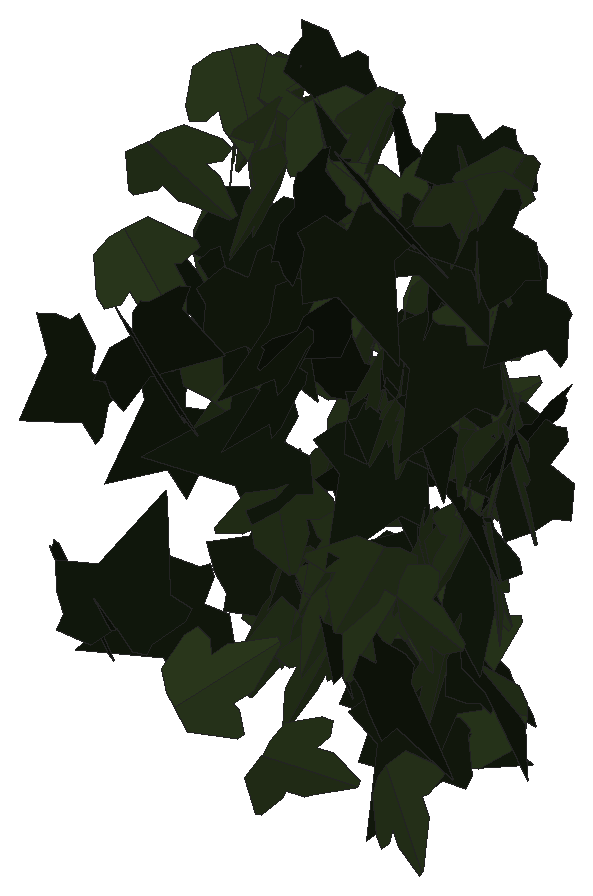
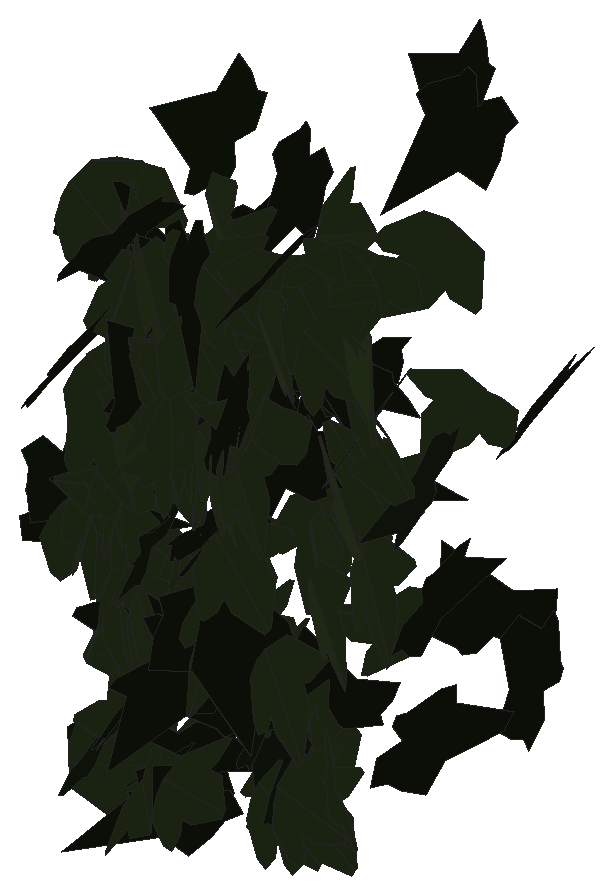
# SketchUp Ruby script. Lengths in inches.
U = 1.inch
M = Sketchup.active_model
def pt(a) = Geom::Point3d.new(a.map { |v| v * U })
def face(e, loops, mat)
  f = e.add_face(loops[0].map { |a| pt(a) })
  loops[1..].each { |l| e.add_face(l.map { |a| pt(a) }).erase! }
  f.material = f.back_material = mat if mat
  f
end
# faces: each face lists its corners as indices into pts; further lists are holes
def faces(e, pts, list, mat = nil) = list.each { |f| face(e, (f[0].is_a?(Array) ? f : [f]).map { |l| l.map { |i| pts[i] } }, mat) }
# xy, xz, yz: faces in a plane at the given z, y or x. An outline is a flat list of corners, or four numbers for a rectangle; further outlines are holes
def ring(l) = l.size == 4 ? [[l[0], l[1]], [l[2], l[1]], [l[2], l[3]], [l[0], l[3]]] : l.each_slice(2).to_a
def flat(e, list, mat, &to3) = list.each { |f| face(e, (f[0].is_a?(Array) ? f : [f]).map { |l| ring(l).map { |u, v| to3.(u, v) } }, mat) }
def xy(e, z, list, mat = nil) = flat(e, list, mat) { |x, y| [x, y, z] }
def xz(e, y, list, mat = nil) = flat(e, list, mat) { |x, z| [x, y, z] }
def yz(e, x, list, mat = nil) = flat(e, list, mat) { |y, z| [x, y, z] }
def lines(e, pts, list) = list.each { |a, b| e.add_line(pt(pts[a]), pt(pts[b])) }
# prism: a flat outline (further loops are holes) pulled along v
def prism(e, loops, v, mat = nil)
  f = face(e, loops, mat); d = Geom::Vector3d.new(v.map { |x| x * U })
  f.pushpull(f.normal.samedirection?(d) ? d.length : -d.length)
end
def box(e, o, s, mat = nil) = prism(e, [[o, [o[0] + s[0], o[1], o[2]], [o[0] + s[0], o[1] + s[1], o[2]], [o[0], o[1] + s[1], o[2]]]], [0, 0, s[2]], mat)
def at(x, y, z, deg = 0) = Geom::Transformation.translation(pt([x, y, z])) * Geom::Transformation.rotation(ORIGIN, Z_AXIS, deg.degrees)
def axes(o, x, y, z) = Geom::Transformation.new([*x, 0, *y, 0, *z, 0, *pt(o).to_a, 1])
def part(name) = M.definitions.add(name)
# library, detail: a bought-in or finely detailed component or shape, given as its bounding box
def library(name, o, s) = part(name).tap { |d| box(d.entities, o, s) }
def detail(e, o, s) = box(e.add_group.entities, o, s)
def put(e, d, t, mat = nil) = e.add_instance(d, t).tap { |i| i.material = mat if mat }
def group(e, t, mat = nil) = e.add_group.tap { |g| g.transformation = t; g.material = mat if mat }.entities
root = M.entities
M.materials.add("efeu1").color = [18, 25, 13]
M.materials.add("efeu2").color = [43, 57, 29]
c1 = part("ivyleaf_9")
p = [[1.54,2.16,1.25],[1.36,2.04,1.19],[-0.21,0.99,0.68],[-0.71,1.11,0.82],[-0.85,0.86,0.67],[-0.8,0.17,0.21],
  [-0.9,-0.01,0.1],[-0.67,-0.16,-0.02],[-0.08,-0.08,-0.05],[-0.03,-0.6,-0.4],[0.65,-0.88,-0.66],[0.83,-0.6,-0.49],
  [1.29,-0.42,-0.43],[1.8125,-0.07,-0.26],[1.21,0.44,0.15]]
faces(c1.entities,p,[[0,1,2,3,4,5,6,7,8,9,10,11,12,13,14]],"efeu1")
c2 = part("ivyleaf_10")
p = [[0,0.5,-0.03],[-0.0625,2.02,-0.43],[-0.19,2.01,-0.46],[-0.54,1.05,-0.29],[-0.52,0.625,-0.18],[-0.83,0.76,-0.28],
  [-1.16,0.64,-0.33],[-1.15,0.33,-0.24],[-0.77,-0.39,0.02],[-0.3,-0.51,0.16],[0.04,-0.48,0.23],[-0.02,2.01,-0.4375],
  [-0.06,2.01,-0.43],[0.04,-0.49,0.23],[0.67,-0.49,0.14],[1.38,0.36,-0.2],[1.375,0.51,-0.24],[0.81,0.65,-0.19],
  [0.62,0.59,-0.15],[0.6,1.09,-0.28],[0.5,1.23,-0.31]]
faces(c2.entities,p,[[0,1,2,3,4,5,6,7,8,9,10],[11,12,0,13,14,15,16,17,18,19,20]],"efeu2")
put(root,c1,axes([16.54,219.83,213.34],[0.188,-0.2735,0.37397],[0.21273,-0.30758,-0.33188],[0.41159,0.28389,0.00071]))
put(root,c1,axes([16.31,219.95,213.48],[-0.01706,0.02207,-0.49922],[-0.18271,0.46465,0.02679],[0.46511,0.18334,-0.00779]))
put(root,c1,axes([14.14,221.85,211.46],[-0.13324,-0.24699,0.41382],[-0.06307,-0.41671,-0.26902],[0.47778,-0.12388,0.07989]))
put(root,c1,axes([14.71,221.64,208.79],[-0.35031,-0.05535,0.35244],[0.34662,0.06414,0.3546],[-0.08447,0.49277,-0.00657]))
put(root,c2,axes([15.83,221.51,208.41],[0.21265,0.07401,-0.44643],[0.30623,0.33963,0.20217],[0.33317,-0.3594,0.09912]))
put(root,c1,axes([13.72,222.1,208.7],[0.32749,-0.0844,-0.36827],[0.3718,-0.01471,0.33399],[-0.06721,-0.4926,0.05313]))
put(root,c1,axes([15.91,222.8,210.83],[-0.10614,-0.16484,-0.45996],[-0.27295,-0.37039,0.19573],[-0.40526,0.29264,-0.01136]))
put(root,c2,axes([16.3,222.34,207.42],[-0.17963,-0.2138,-0.41476],[0.26858,0.31605,-0.27924],[0.38157,-0.32311,0.0013]))
put(root,c1,axes([16.1875,222.73,211.82],[-0.42076,0.25909,-0.07637],[0.06401,-0.0417,-0.49413],[-0.26241,-0.4256,0.00192]))
put(root,c1,axes([17.07,222.87,214.14],[0.26386,-0.28378,0.31599],[0.24447,-0.20272,-0.38619],[0.3473,0.35829,0.03177]))
put(root,c1,axes([14.57,223.16,208.26],[-0.02002,-0.2401,-0.43812],[0.05042,-0.43721,0.2373],[-0.49705,-0.03468,0.04172]))
put(root,c2,axes([15.97,222.73,210.17],[-0.31787,-0.37955,-0.06999],[0.04483,0.05375,-0.49508],[0.38334,-0.32102,-0.00014]))
put(root,c1,axes([16.1875,222.8,212.32],[-0.44206,0.23135,-0.0325],[0.02778,-0.01702,-0.49894],[-0.23197,-0.44293,0.00219]))
put(root,c2,axes([15.55,223.13,213.67],[0.09818,-0.17269,0.45884],[0.19718,-0.41453,-0.19821],[0.44886,0.21987,-0.01329]))
put(root,c1,axes([16.42,222.47,213.93],[0.01627,0.04836,-0.49739],[-0.34136,0.36454,0.02428],[0.36498,0.33878,0.04487]))
put(root,c2,axes([14.46,222.76,213.76],[-0.37573,-0.13553,-0.30077],[0.27848,0.11408,-0.39929],[0.17685,-0.46757,-0.01024]))
put(root,c2,axes([17.45,222.82,207.26],[-0.04018,0.49014,0.09025],[-0.00647,0.09003,-0.49179],[-0.49834,-0.04069,-0.00089]))
put(root,c2,axes([16.96,223.09,209.67],[-0.30127,-0.34549,0.19969],[-0.1342,-0.14791,-0.45838],[0.3758,-0.32979,-0.00361]))
put(root,c1,axes([16.69,222.99,213.47],[0.08596,-0.42301,-0.25234],[-0.04112,0.24909,-0.43158],[0.49084,0.09495,0.00803]))
put(root,c1,axes([17.03,223.07,208.42],[0.01122,-0.01107,-0.49975],[0.4804,0.13839,0.00772],[0.13815,-0.48034,0.01374]))
put(root,c2,axes([13.87,222.96,212.3],[0.34879,0.20575,0.29328],[0.25683,0.14176,-0.4049],[-0.24976,0.4331,-0.00679]))
put(root,c1,axes([16.27,222.72,212.32],[0.17672,0.45514,0.10779],[0.03908,0.10045,-0.48824],[-0.46609,0.18099,-0.00007]))
put(root,c2,axes([17.36,223.23,209.22],[-0.0175,0.01973,-0.4993],[0.4142,-0.27891,-0.02554],[-0.27953,-0.41451,-0.00658]))
put(root,c1,axes([14.02,223.56,210.21],[0.1056,-0.1992,-0.44628],[0.2361,-0.37897,0.22502],[-0.42791,-0.25826,0.01403]))
put(root,c1,axes([15.28,223.13,212.36],[0.07663,-0.36845,-0.3292],[-0.01661,0.33103,-0.37436],[0.49381,0.06831,0.03849]))
put(root,c2,axes([15.94,223.64,208.67],[-0.04075,-0.22604,0.44412],[0.24144,-0.39877,-0.1808],[0.43594,0.19972,0.14165]))
put(root,c2,axes([14.82,223.25,210.9],[-0.34636,-0.2454,0.26422],[0.21472,0.15399,0.42448],[-0.28971,0.40751,-0.00129]))
put(root,c1,axes([14.78,223.75,211.84],[-0.00361,-0.39451,0.30717],[0.01593,-0.30711,-0.39425],[0.49973,0.00693,0.01479]))
put(root,c2,axes([16.75,223.67,208.89],[-0.22085,-0.36156,0.26551],[-0.06302,-0.268,-0.41738],[0.44413,-0.21782,0.0728]))
put(root,c2,axes([15.16,223.83,208.27],[-0.00661,0.04642,-0.4978],[0.01534,-0.49759,-0.04661],[-0.49972,-0.01588,0.00515]))
put(root,c1,axes([16.53,223.91,210.38],[-0.20079,-0.42052,0.18123],[-0.05561,-0.17403,-0.46543],[0.45452,-0.20707,0.02312]))
put(root,c1,axes([15.78,223.91,208.3125],[0.05501,-0.30494,0.39241],[0.09586,-0.38088,-0.30942],[0.48763,0.10928,0.01656]))
put(root,c2,axes([15.91,223.93,209.26],[0.00645,-0.24716,0.43459],[0.1418,-0.41587,-0.23862],[0.47943,0.12633,0.06473]))
put(root,c1,axes([17.02,223.9375,207.4],[-0.22715,-0.42794,0.12358],[-0.04293,-0.11704,-0.48421],[0.44335,-0.23059,0.01643]))
put(root,c1,axes([14.89,223.78,212.7],[-0.33845,-0.23923,-0.27968],[0.25203,0.12625,-0.41297],[0.26821,-0.42051,0.03513]))
put(root,c1,axes([15.68,223.75,211.09],[0.47176,0.1266,0.10682],[-0.1062,-0.01625,0.48832],[0.12712,-0.48343,0.01156]))
put(root,c2,axes([15.4375,223.77,208.64],[-0.28687,-0.01127,0.40937],[0.4088,-0.03754,0.28544],[0.0243,0.49846,0.03075]))
put(root,c2,axes([17.33,223.74,208.49],[0.0812,-0.492,-0.03671],[-0.00668,0.0361,-0.49865],[0.49332,0.08147,-0.00071]))
put(root,c1,axes([13.8,223.76,211.75],[0.35493,-0.3521,-0.00697],[-0.00262,0.00726,-0.49994],[0.35216,0.35492,0.0033]))
put(root,c2,axes([15.27,223.71,210.49],[0.21687,-0.43763,-0.107],[-0.03337,0.10282,-0.48817],[0.44928,0.21888,0.01539]))
put(root,c1,axes([17.34,224.07,211.875],[-0.22181,-0.42481,0.14259],[-0.03553,-0.14193,-0.47811],[0.4467,-0.22224,0.03277]))
put(root,c1,axes([15.31,223.6,208.53],[-0.41354,-0.09877,0.26311],[0.25548,0.06293,0.42517],[-0.11711,0.48609,-0.00158]))
put(root,c2,axes([16.62,223.95,213.23],[0.16113,0.33211,0.33726],[-0.15927,-0.29745,0.369],[0.44572,-0.22634,0.00994]))
put(root,c2,axes([14.49,223.86,210.53],[0.07881,-0.49369,0.00737],[-0.00157,-0.00771,-0.49994],[0.49375,0.07878,-0.00276]))
put(root,c2,axes([16.79,223.65,211.27],[0.08838,-0.39522,-0.29325],[-0.05077,0.28902,-0.40483],[0.4895,0.10134,0.01096]))
put(root,c1,axes([16.79,224.14,211.12],[0.11425,-0.42028,0.24558],[0.10259,-0.2258,-0.43416],[0.47584,0.14959,0.03464]))
put(root,c2,axes([16.05,223.84,212.78],[-0.47911,-0.14242,-0.01293],[0.01239,0.00368,-0.49983],[0.14247,-0.47927,0]))
put(root,c1,axes([15.35,224.19,207.96],[0.15502,-0.30113,0.36782],[0.16247,-0.33003,-0.33865],[0.44674,0.22451,-0.00447]))
put(root,c1,axes([16.78,224.04,207.91],[-0.28341,-0.33523,-0.23938],[0.14955,0.187,-0.43894],[0.38382,-0.32039,-0.00573]))
put(root,c2,axes([16.27,224.0625,214.09],[0.27368,-0.40287,0.11311],[0.05385,-0.10012,-0.4869],[0.41497,0.27869,-0.01141]))
put(root,c2,axes([15.48,224.16,207.6875],[-0.00254,-0.42944,0.25608],[0.00996,-0.25608,-0.42933],[0.49989,0.00292,0.00985]))
put(root,c2,axes([16.97,223.78,209.51],[0.10993,-0.41141,-0.26203],[0.00819,0.27012,-0.42067],[0.4877,0.0882,0.06613]))
put(root,c1,axes([17.93,224.05,213.53],[-0.09306,-0.0759,-0.48536],[-0.37124,-0.31267,0.12007],[-0.32174,0.38272,0.00184]))
put(root,c2,axes([16.79,224.125,211.2],[0.06298,-0.47064,0.15663],[0.04524,-0.15178,-0.47425],[0.49395,0.07391,0.02346]))
put(root,c2,axes([17.6,223.9,213.88],[-0.37441,-0.30402,-0.13187],[0.10063,0.08527,-0.48229],[0.31574,-0.38768,-0.00267]))
put(root,c2,axes([14.04,224.06,211.85],[0.3603,-0.16451,-0.30515],[0.28409,-0.11212,0.39588],[-0.19868,-0.45866,0.01268]))
put(root,c2,axes([14.99,224.29,207.85],[-0.05518,-0.41312,0.2762],[-0.01421,-0.27647,-0.41637],[0.49674,-0.0538,0.01877]))
put(root,c1,axes([16.17,224.24,210.54],[0.16625,-0.47101,0.02255],[0.00781,-0.02116,-0.49949],[0.47149,0.16643,0.00032]))
put(root,c1,axes([16.95,224.09,213.33],[-0.1368,-0.29957,-0.37623],[0.22733,0.30442,-0.32504],[0.4238,-0.25998,0.05291]))
put(root,c2,axes([14.34,224.02,214.11],[0.40785,0.2367,0.16624],[0.13838,0.09267,-0.47145],[-0.25399,0.43057,0.01008]))
put(root,c1,axes([16.0625,224.01,208.53],[-0.16197,0.03552,0.4717],[0.44777,-0.14927,0.16499],[0.15254,0.47587,0.01655]))
put(root,c2,axes([17.28,224.32,213.3],[-0.11656,0.21827,-0.43448],[0.20482,-0.38317,-0.24744],[-0.44098,-0.23567,-0.00008]))
put(root,c1,axes([16.96,224.32,210.14],[0.23966,-0.36897,0.23753],[0.13433,-0.19597,-0.43995],[0.41775,0.27469,0.0052]))
put(root,c2,axes([16.28,224.15,211.44],[0.11995,-0.48224,-0.05532],[-0.01963,0.05212,-0.49689],[0.485,0.12137,-0.00643]))
put(root,c2,axes([17.55,224.3,209.47],[-0.17466,0.31822,-0.34384],[0.15503,-0.30703,-0.3629],[-0.44211,-0.23338,0.00859]))
put(root,c2,axes([16.39,223.77,212.96],[0.04582,-0.0815,-0.49118],[0.20427,0.45291,-0.0561],[0.45406,-0.19553,0.0748]))
put(root,c2,axes([14.5,224.15,213.92],[-0.17611,-0.01283,-0.46778],[0.46275,-0.07911,-0.17205],[-0.0696,-0.49354,0.03974]))
put(root,c2,axes([17.66,224.44,213.92],[-0.05707,-0.41098,0.27899],[-0.01494,-0.27928,-0.41446],[0.49651,-0.05564,0.01959]))
put(root,c2,axes([14.81,224.38,213.63],[-0.07339,-0.46596,0.16582],[-0.02776,-0.16349,-0.4717],[0.4938,-0.07844,-0.00187]))
put(root,c2,axes([16.9,224.34,211.72],[-0.0399,-0.48844,0.09917],[-0.00314,-0.09924,-0.49004],[0.4984,-0.03973,0.00485]))
put(root,c1,axes([16.84,224.12,211.98],[0.06335,-0.34112,-0.36004],[-0.05462,0.35596,-0.34686],[0.49295,0.08328,0.00784]))
put(root,c1,axes([16.64,223.97,207.29],[0.18892,-0.07851,-0.45623],[0.04344,0.49359,-0.06695],[0.46089,-0.01434,0.19332]))
put(root,c2,axes([17.06,224.59,209.51],[0.05222,-0.32914,0.37274],[0.0779,-0.36475,-0.333],[0.49112,0.09286,0.01319]))
put(root,c1,axes([17.27,224.5,208.05],[0.04101,-0.49823,0.00941],[0.02119,0.01118,0.49943],[-0.49786,-0.04057,0.02203]))
put(root,c2,axes([17.58,224.39,207.52],[-0.02311,0.00636,-0.49943],[-0.49243,-0.08394,0.02171],[-0.08357,0.49286,0.01014]))
put(root,c2,axes([16.89,224.41,209.41],[0.08213,-0.48218,0.1037],[0.01679,-0.10234,-0.48913],[0.49292,0.08383,-0.00062]))
put(root,c2,axes([17.39,224.04,213.64],[0.10619,-0.20016,-0.44571],[-0.23619,0.37825,-0.22614],[0.42771,0.25857,-0.01421]))
put(root,c1,axes([17.37,224.54,207.88],[0.17724,-0.40596,0.23191],[0.11313,-0.2034,-0.44253],[0.45364,0.20934,0.01975]))
put(root,c2,axes([17.39,224.55,212.08],[-0.18514,-0.37792,0.27],[0.02022,-0.29694,-0.40177],[0.46402,-0.13785,0.12523]))
put(root,c2,axes([16.63,224.41,212.02],[0.01279,0.46453,-0.18451],[-0.00164,-0.18453,-0.4647],[-0.49983,0.01249,-0.0032]))
put(root,c2,axes([16.2,224.52,212.9],[-0.19655,-0.40359,0.22019],[-0.04582,-0.22108,-0.44612],[0.45746,-0.19555,0.04992]))
put(root,c2,axes([14.82,224.66,208.16],[0.04436,-0.34675,0.35749],[0.07048,-0.35092,-0.34912],[0.49302,0.08136,0.01775]))
put(root,c1,axes([17,224.44,209.3125],[-0.27512,-0.23506,-0.34504],[0.27351,0.21073,-0.36164],[0.31543,-0.38774,0.01264]))
put(root,c2,axes([15.38,224.25,213.82],[0.25809,0.39595,0.16313],[0.08886,0.13681,-0.47264],[-0.41892,0.27296,0.00025]))
put(root,c2,axes([17.16,224.28,208.15],[0.24175,0.43611,-0.0369],[0.01376,0.03456,0.49861],[0.43745,-0.2421,0.00471]))
put(root,c2,axes([14.3125,224.6,208.39],[0.26943,-0.15732,0.39071],[0.3506,-0.17328,-0.31154],[0.23343,0.44184,0.01694]))
put(root,c2,axes([17.53,224.6,210.89],[0.32597,-0.32043,0.20265],[0.13349,-0.15314,-0.45687],[0.35485,0.35196,-0.01428]))
put(root,c2,axes([15.48,224.24,212.05],[0.26998,0.32125,0.27186],[0.15316,0.22585,-0.41897],[-0.39199,0.3095,0.02354]))
put(root,c2,axes([15.8125,224.56,211.49],[0.16668,-0.46344,0.08626],[0.03886,-0.07767,-0.4924],[0.4698,0.17085,0.01013]))
put(root,c2,axes([13.84,224.77,213.08],[-0.04421,-0.12954,-0.4809],[0.18844,-0.45125,0.10423],[-0.46102,-0.17203,0.08872]))
put(root,c2,axes([17.01,224.51,213.13],[-0.314,0.19098,-0.33901],[0.29297,-0.17065,-0.36749],[-0.25607,-0.42942,-0.00474]))
put(root,c2,axes([16.74,224.82,211.3],[-0.04304,-0.15664,-0.47288],[0.06777,-0.47207,0.1502],[-0.49351,-0.05117,0.06187]))
put(root,c1,axes([17.9,224.71,210.43],[-0.16071,-0.21905,-0.41975],[-0.24688,-0.33947,0.27168],[-0.40401,0.29458,0.00095]))
put(root,c2,axes([15.71,224.75,213.8125],[0.03813,-0.40074,0.29657],[0.03428,-0.29463,-0.40252],[0.49736,0.05102,0.00501]))
put(root,c2,axes([15.64,224.7,210.67],[-0.13434,-0.42773,0.22137],[-0.01167,-0.22686,-0.44542],[0.48147,-0.12484,0.05096]))
put(root,c2,axes([14.52,224.61,210.52],[0.20609,-0.45254,0.05229],[0.01754,-0.04946,-0.49724],[0.45521,0.20679,-0.00451]))
put(root,c2,axes([17.21,224.22,210.84],[0.14068,-0.23101,-0.42053],[-0.02785,0.43356,-0.24749],[0.47899,0.09306,0.10911]))
put(root,c2,axes([17.02,224.82,210.12],[-0.04804,0.22406,-0.4444],[0.07091,-0.43883,-0.22892],[-0.49261,-0.08502,0.01039]))
put(root,c1,axes([17.05,224.75,213.89],[-0.02766,-0.49852,-0.02667],[0.00614,0.02637,-0.49927],[0.4992,-0.02795,0.00466]))
put(root,c1,axes([16.4,224.39,213.8],[0.2313,0.01374,-0.44307],[-0.44326,0.00245,-0.23132],[-0.00419,0.49981,0.01331]))
put(root,c2,axes([15.06,224.66,209.51],[0.02348,-0.4938,0.07491],[-0.00275,-0.07512,-0.49432],[0.49944,0.0228,-0.00624]))
put(root,c2,axes([17.56,224.6,210.56],[-0.28506,0.34376,-0.22487],[0.14886,-0.16866,-0.44653],[-0.38286,-0.32153,-0.00619]))
put(root,c2,axes([16.01,224.38,209.7],[-0.08304,-0.40574,-0.28014],[0.04267,0.2771,-0.414],[0.49121,-0.09266,-0.0114]))
put(root,c2,axes([16.76,224.7,207.62],[-0.0478,0.42388,-0.26085],[0.02938,-0.25919,-0.42656],[-0.49684,-0.05611,-0.00013]))
put(root,c2,axes([15.58,224.22,212.36],[-0.09229,0.12614,0.47494],[-0.2667,0.39303,-0.15621],[-0.41274,-0.28217,-0.00527]))
put(root,c2,axes([16.92,224.67,209.12],[0.21837,-0.06624,0.44489],[0.44237,-0.05787,-0.22574],[0.0814,0.4922,0.03333]))
put(root,c1,axes([17.86,224.53,210.9375],[-0.19367,0.42641,-0.17512],[0.07455,-0.15847,-0.46832],[-0.4549,-0.20751,-0.0022]))
put(root,c1,axes([15.49,224.87,212.13],[0.06542,-0.1538,0.47124],[0.16039,-0.44319,-0.16691],[0.46904,0.173,-0.00865]))
put(root,c1,axes([15.91,224.49,209.84],[0.10396,0.41742,-0.25487],[-0.07956,-0.24265,-0.42987],[-0.48256,0.12994,0.01597]))
put(root,c2,axes([17.42,224.84,210.52],[-0.24778,-0.28274,0.32965],[-0.0725,-0.34727,-0.35235],[0.42819,-0.2224,0.13109]))
put(root,c2,axes([16.1,224.91,207.9375],[-0.09123,-0.30004,0.38942],[0.1311,-0.39658,-0.27484],[0.4738,0.05196,0.15103]))
put(root,c2,axes([15.52,224.68,211.74],[0.06679,-0.4928,0.05179],[0.00239,-0.05194,-0.49729],[0.49551,0.06668,-0.00458]))
put(root,c2,axes([16.67,224.65,213.51],[0.15549,-0.47501,0.01372],[0.00428,-0.01303,-0.49981],[0.47519,0.15555,0.00001]))
put(root,c1,axes([15.07,224.87,214.125],[0.04483,-0.48055,0.13063],[0.02579,-0.12875,-0.48245],[0.49732,0.05,0.01324]))
put(root,c2,axes([15.0625,224.75,213.47],[0.28704,-0.38228,0.14653],[0.08464,-0.11968,-0.47803],[0.40055,0.29924,-0.00399]))
put(root,c2,axes([17.64,224.6,210.83],[-0.39573,0.30554,0.00649],[0.00484,-0.00435,0.49996],[0.30557,0.39576,0.00048]))
put(root,c2,axes([16.8125,224.64,212.52],[0.47717,-0.05408,-0.13924],[-0.13859,0.01363,-0.48022],[0.05574,0.49688,-0.00198]))
put(root,c2,axes([14.1,224.71,211.46],[0.29944,-0.32703,-0.23105],[0.16836,-0.15894,0.44316],[-0.36331,-0.3432,0.01493]))
put(root,c1,axes([16.97,224.38,211.97],[-0.03012,-0.20956,0.45296],[0.20399,0.40899,0.20278],[-0.4555,0.19701,0.06086]))
put(root,c2,axes([17.38,224.58,210.68],[-0.08761,-0.4815,-0.10237],[0.02397,0.09968,-0.48938],[0.49168,-0.09065,0.00562]))
put(root,c1,axes([16.36,224.52,209.01],[0.00477,-0.31867,-0.38526],[0.03569,0.38451,-0.31761],[0.4987,-0.02447,0.02641]))
put(root,c2,axes([17.16,224.73,211.74],[-0.21754,-0.43308,0.12297],[-0.02872,-0.12295,-0.4838],[0.44928,-0.21755,0.02862]))
put(root,c2,axes([14.29,224.9,213.62],[-0.02176,-0.3867,0.31621],[0.05039,-0.31659,-0.38371],[0.49698,0.01516,0.05275]))
put(root,c1,axes([17.63,225.03,212.21],[-0.11443,-0.3282,0.35943],[-0.03678,-0.36234,-0.34257],[0.48534,-0.10484,0.05878]))
put(root,c2,axes([16.5,224.48,211.4],[0.20788,0.44176,-0.10785],[0.01739,0.11078,0.48726],[0.4544,-0.20634,0.03069]))
put(root,c2,axes([16.98,224.33,210.75],[0.10124,0.11173,-0.47672],[0.33877,0.3355,0.15058],[0.35353,-0.35349,-0.00778]))
